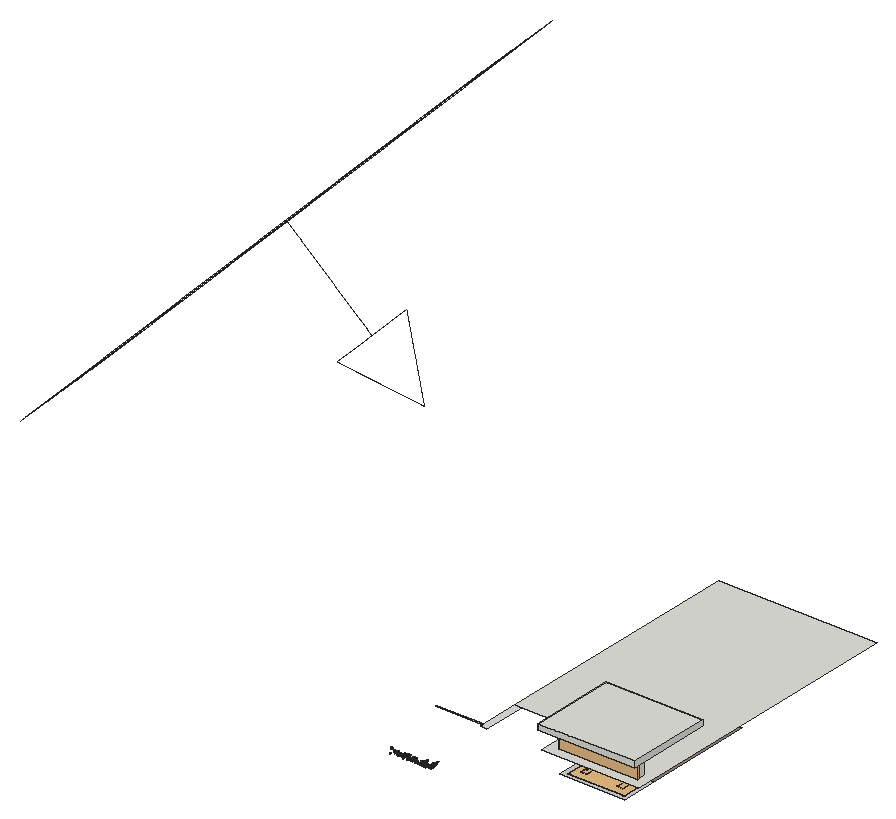
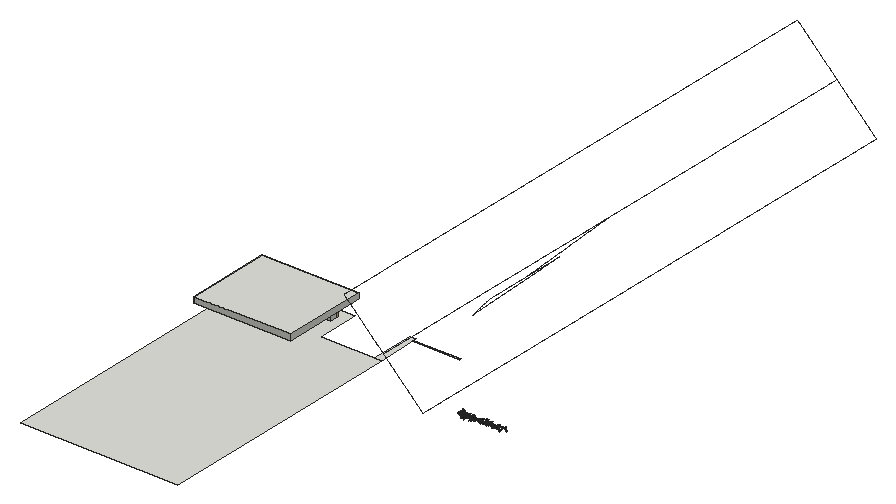
# SketchUp Ruby script. Lengths in inches.
U = 1.inch
M = Sketchup.active_model
def pt(a) = Geom::Point3d.new(a.map { |v| v * U })
def face(e, loops, mat)
  f = e.add_face(loops[0].map { |a| pt(a) })
  loops[1..].each { |l| e.add_face(l.map { |a| pt(a) }).erase! }
  f.material = f.back_material = mat if mat
  f
end
# faces: each face lists its corners as indices into pts; further lists are holes
def faces(e, pts, list, mat = nil) = list.each { |f| face(e, (f[0].is_a?(Array) ? f : [f]).map { |l| l.map { |i| pts[i] } }, mat) }
# xy, xz, yz: faces in a plane at the given z, y or x. An outline is a flat list of corners, or four numbers for a rectangle; further outlines are holes
def ring(l) = l.size == 4 ? [[l[0], l[1]], [l[2], l[1]], [l[2], l[3]], [l[0], l[3]]] : l.each_slice(2).to_a
def flat(e, list, mat, &to3) = list.each { |f| face(e, (f[0].is_a?(Array) ? f : [f]).map { |l| ring(l).map { |u, v| to3.(u, v) } }, mat) }
def xy(e, z, list, mat = nil) = flat(e, list, mat) { |x, y| [x, y, z] }
def xz(e, y, list, mat = nil) = flat(e, list, mat) { |x, z| [x, y, z] }
def yz(e, x, list, mat = nil) = flat(e, list, mat) { |y, z| [x, y, z] }
def lines(e, pts, list) = list.each { |a, b| e.add_line(pt(pts[a]), pt(pts[b])) }
# prism: a flat outline (further loops are holes) pulled along v
def prism(e, loops, v, mat = nil)
  f = face(e, loops, mat); d = Geom::Vector3d.new(v.map { |x| x * U })
  f.pushpull(f.normal.samedirection?(d) ? d.length : -d.length)
end
def box(e, o, s, mat = nil) = prism(e, [[o, [o[0] + s[0], o[1], o[2]], [o[0] + s[0], o[1] + s[1], o[2]], [o[0], o[1] + s[1], o[2]]]], [0, 0, s[2]], mat)
def at(x, y, z, deg = 0) = Geom::Transformation.translation(pt([x, y, z])) * Geom::Transformation.rotation(ORIGIN, Z_AXIS, deg.degrees)
def axes(o, x, y, z) = Geom::Transformation.new([*x, 0, *y, 0, *z, 0, *pt(o).to_a, 1])
def part(name) = M.definitions.add(name)
# library, detail: a bought-in or finely detailed component or shape, given as its bounding box
def library(name, o, s) = part(name).tap { |d| box(d.entities, o, s) }
def detail(e, o, s) = box(e.add_group.entities, o, s)
def put(e, d, t, mat = nil) = e.add_instance(d, t).tap { |i| i.material = mat if mat }
def group(e, t, mat = nil) = e.add_group.tap { |g| g.transformation = t; g.material = mat if mat }.entities
root = M.entities
M.materials.add("Concrete White 02 100cm").color = [209, 209, 209]
M.materials.add("Heather_Band").color = [140, 131, 120]
M.materials.add("efeu1").color = [18, 25, 13]
c1 = part("ivyleaf_9")
p = [[1.54,2.16,1.25],[1.36,2.04,1.19],[-0.21,0.99,0.68],[-0.71,1.11,0.82],[-0.85,0.86,0.67],[-0.8,0.17,0.21],
  [-0.9,-0.01,0.1],[-0.67,-0.16,-0.02],[-0.08,-0.08,-0.05],[-0.03,-0.6,-0.4],[0.65,-0.88,-0.66],[0.83,-0.6,-0.49],
  [1.29,-0.42,-0.43],[1.8125,-0.07,-0.26],[1.21,0.44,0.15]]
faces(c1.entities,p,[[0,1,2,3,4,5,6,7,8,9,10,11,12,13,14]],"efeu1")
c2 = library("Tlon Light 450 Ceiling 152 006",[-8.86,-8.86,-3.78],[17.72,17.72,3.56])
c3 = part("Tlon Cubo 860 Ceiling 152 005")
xy(c3.entities,-3.04,[[-16.54,-16.54,-16.54,16.54,16.54,-16.54],[16.54,-16.54,-16.54,16.54,16.54,16.54]])
xy(c3.entities,0,[[-16.93,-16.93,16.93,-16.93,-16.93,16.93],[16.93,-16.93,16.93,16.93,-16.93,16.93]])
xz(c3.entities,-16.93,[[-16.93,-3.79,16.93,-3.79,-16.93,0],[16.93,-3.79,16.93,0,-16.93,0]])
xz(c3.entities,-16.3,[[-16.3,-3.66,-16.3,-3.24,16.3,-3.24],[-16.3,-3.66,16.3,-3.24,16.3,-3.66]])
xz(c3.entities,16.3,[[-16.3,-3.66,16.3,-3.24,-16.3,-3.24],[-16.3,-3.66,16.3,-3.66,16.3,-3.24]])
xz(c3.entities,16.93,[[-16.93,-3.79,-16.93,0,16.93,0],[-16.93,-3.79,16.93,0,16.93,-3.79]])
yz(c3.entities,-16.93,[[-16.93,-3.79,-16.93,0,16.93,0],[-16.93,-3.79,16.93,0,16.93,-3.79]])
yz(c3.entities,-16.3,[[-16.3,-3.66,16.3,-3.66,-16.3,-3.24],[16.3,-3.66,16.3,-3.24,-16.3,-3.24]])
yz(c3.entities,16.3,[[-16.3,-3.66,-16.3,-3.24,16.3,-3.66],[16.3,-3.66,-16.3,-3.24,16.3,-3.24]])
yz(c3.entities,16.93,[[-16.93,-3.79,16.93,-3.79,-16.93,0],[16.93,-3.79,16.93,0,-16.93,0]])
p = [[-16.93,-16.93,-3.79],[-16.93,16.93,-3.79],[-16.3,16.3,-3.66],[-16.3,-16.3,-3.66],[16.93,-16.93,-3.79],[16.3,-16.3,-3.66],
  [16.93,16.93,-3.79],[16.3,16.3,-3.66]]
faces(c3.entities,p,[[0,1,2],[2,3,0],[4,0,3],[3,5,4],[6,4,5],[5,7,6],[2,1,6],[6,7,2]])
c4 = library("Group\#2",[-0.5,-0.5,-0.1],[76.5625,123.26,0.2])
c5 = library("Group\#11",[-0.5,-0.5,-0.1],[80.125,38.25,0.2])
c6 = library("Wall Panel 104-26",[-34.24,-2.8,0],[68.48,2.8,108.01])
c7 = part("Group418\#1")
p = [[0,0,0],[0,0,-140.58],[-66.03,0,-140.58],[429.86,-25.26,0],[-429.86,-25.26,0],[429.86,25.26,0],
  [429.86,0,0],[-429.86,25.26,0],[66.03,0,-140.58],[-429.86,0,0],[0,0,-227.5625]]
lines(c7.entities,p,[[0,1],[1,2],[3,4],[5,6],[7,5],[1,8],[9,0],[0,6],[8,10],[4,9],[6,3],[2,10],
  [9,7]])
c8 = part("Rectangle Light\#1")
put(c8.entities,c7,at(0,0,0))
xy(root,316.43,[[[245.01,223.4375,337.3,273.83],[252.75,229.09,331.875,266.34]],[254.75,231.09,329.875,264.34]],"Concrete White 02 100cm")
xy(root,316.43,[[[245.01,273.83,337.3,430.75],[253.2,286.86,328.77,409.125]],[255.2,288.86,326.77,407.125]],"Heather_Band")
xy(root,337.75,[[133.125,223.4375,142.16,284.3125],[[219.21,223.4375,356.8125,223.4375,356.8125,643.9375,133.125,643.9375,133.125,284.3125,219.21,284.3125],[232.57,240.26,343.51,249.58]],[66.5625,227.3125,133.125,229.125]])
xy(root,360.8,[[213.82,224.2,213.82,344.45,350.32,344.45,350.32,249.58,232.57,249.58,232.57,240.26,350.32,240.26,350.32,224.2],[232.57,240.26,343.51,249.58],[343.51,240.26,350.32,249.58]])
xy(root,369,[[213.82,224.2,350.32,344.45]])
xz(root,224.2,[[213.82,360.8,350.32,369]])
xz(root,240.26,[[232.57,337.75,343.51,360.8]])
xz(root,249.58,[[232.57,337.75,343.51,360.8]])
xz(root,344.45,[[213.82,360.8,350.32,369]])
yz(root,213.82,[[224.2,360.8,344.45,369]])
yz(root,232.57,[[240.26,337.75,249.58,360.8]])
yz(root,343.51,[[240.26,337.75,249.58,360.8]])
yz(root,350.32,[[224.2,360.8,344.45,369]])
put(root,c1,axes([54.86,220.23,262.29],[-0.42599,-0.23908,0.10667],[-0.08419,-0.0678,-0.48818],[0.24789,-0.43387,0.01751]))
put(root,c1,axes([54.96,223.33,262.27],[-0.42097,0.2695,0.0124],[-0.06704,-0.08224,-0.48861],[-0.26132,-0.41304,0.10537]))
put(root,c1,axes([44.03,219.59,262.4],[0.30234,-0.38809,-0.08932],[-0.02728,0.0917,-0.49076],[0.3973,0.30163,0.03428]))
put(root,c1,axes([64.83,220.53,262.52],[0.41955,-0.2121,-0.17026],[-0.05677,0.2378,-0.43615],[0.26599,0.38531,0.17546]))
put(root,c1,axes([27.72,218.6,262.27],[-0.41659,-0.27335,0.04161],[-0.03507,-0.0224,-0.49827],[0.27426,-0.41807,-0.00051]))
put(root,c1,axes([61.34,220.32,262.58],[0.1176,-0.43666,-0.2133],[0.00401,0.22032,-0.44883],[0.48596,0.10386,0.05533]))
put(root,c1,axes([53.86,220.5,262.4],[-0.38441,0.31571,-0.05054],[0.02059,-0.05442,-0.4966],[-0.31907,-0.38388,0.02884]))
put(root,c1,axes([34.49,220.18,262.66],[0.1015,-0.41881,-0.25356],[0.06389,0.26807,-0.4172],[0.4854,0.05229,0.10793]))
put(root,c1,axes([62.25,220.75,262.43],[0.28877,-0.40492,-0.05146],[0.01714,0.07502,-0.49404],[0.40782,0.28357,0.05721]))
put(root,c1,axes([54.6875,218.44,262.05],[0.04231,-0.15687,0.47286],[0.35975,-0.31869,-0.13791],[0.34466,0.35189,0.08591]))
put(root,c1,axes([64.3,220.32,262.65],[-0.06335,-0.43846,-0.23183],[0.04191,0.22814,-0.44294],[0.4942,-0.07555,0.00785]))
put(root,c1,axes([16.375,220.87,262.39],[0.02361,0.49902,-0.02055],[-0.00029,-0.02056,-0.49958],[-0.49944,0.0236,-0.00068]))
put(root,c1,axes([42.61,220.58,262.42],[0.44072,-0.22677,0.06591],[0.05993,-0.02758,-0.49563],[0.22842,0.44476,0.00287]))
put(root,c1,axes([51.43,220.61,262.45],[-0.04152,-0.48791,0.10112],[-0.01245,-0.10042,-0.48965],[0.49812,-0.04318,-0.00381]))
put(root,c1,axes([62.4,220.6875,262.71],[0.00392,-0.30471,-0.39641],[0.18464,0.36928,-0.28203],[0.46464,-0.14417,0.11542]))
put(root,c1,axes([27.24,219.85,262.5],[-0.41595,0.06259,0.27031],[-0.27588,-0.04138,-0.41495],[-0.02957,-0.49434,0.06895]))
put(root,c1,axes([62.33,220.75,262.4],[0.00894,-0.49992,0.00077],[-0.00005,-0.00077,-0.5],[0.49992,0.00894,-0.00006]))
put(root,c1,axes([32.43,219.17,262.8],[0.22625,-0.3949,-0.20703],[-0.01221,0.22658,-0.44555],[0.44571,0.20667,0.09288]))
put(root,c1,axes([54.54,220.27,262.72],[-0.21236,0.04329,-0.45059],[0.39361,-0.22814,-0.20742],[-0.22355,-0.44281,0.06282]))
put(root,c1,axes([26.86,220.45,262.53],[-0.14827,-0.47751,0.00136],[0.00832,-0.00401,-0.49991],[0.47744,-0.14822,0.00913]))
put(root,c1,axes([63.24,220.27,262.65],[0.13031,0.42767,0.22387],[-0.04054,0.24076,-0.43634],[-0.48102,0.09557,0.09742]))
put(root,c1,axes([52.2,219.52,262.55],[-0.1899,0.28378,0.36525],[-0.22412,0.28893,-0.34101],[-0.40461,-0.29323,0.01747]))
put(root,c1,axes([44.57,218.84,262.68],[-0.23037,-0.41187,0.1652],[-0.02076,-0.17593,-0.46757],[0.44328,-0.22229,0.06396]))
put(root,c1,axes([51.34,219.01,262.74],[-0.26364,-0.41336,0.09811],[-0.00422,-0.11291,-0.48707],[0.42482,-0.25765,0.05605]))
put(root,c1,axes([55.45,222.27,262.38],[0.19075,-0.44838,0.11209],[0.43896,0.13781,-0.19575],[0.14465,0.17309,0.44622]))
put(root,c1,axes([62.76,220.68,262.04],[0.00862,-0.49987,-0.00733],[-0.0052,-0.00742,0.49992],[-0.4999,-0.00854,-0.00532]))
put(root,c1,axes([65.45,220.93,262.85],[-0.32857,-0.36504,-0.09375],[0.09576,0.03944,-0.48916],[0.36452,-0.3394,0.044]))
put(root,c1,axes([24.79,220.5,262.8125],[-0.39253,-0.27217,0.14781],[-0.03644,-0.19638,-0.45837],[0.30756,-0.37062,0.13434]))
put(root,c1,axes([59.54,220.23,263.04],[0.18927,-0.36787,-0.28079],[-0.05174,0.28465,-0.4078],[0.45989,0.18342,0.06968]))
put(root,c1,axes([25.62,220.68,262.78],[-0.14463,-0.46314,0.12077],[0.00539,-0.12773,-0.48338],[0.4786,-0.13852,0.04194]))
put(root,c1,axes([50.69,221.84,262.58],[-0.09558,-0.47416,0.12664],[0.38768,-0.15206,-0.27673],[0.30094,0.04529,0.39671]))
put(root,c1,axes([45.11,219.73,262.8125],[-0.23768,-0.3743,0.2311],[-0.05756,-0.23395,-0.43812],[0.43611,-0.23487,0.06812]))
put(root,c1,axes([59.52,219.48,262.73],[-0.28352,-0.41013,0.03755],[-0.01761,-0.03347,-0.49857],[0.41147,-0.28403,0.00454]))
put(root,c1,axes([56.01,220.41,262.85],[-0.32635,-0.35473,0.13289],[0.00327,-0.17803,-0.46722],[0.37879,-0.30409,0.11852]))
put(root,c1,axes([54.41,220.22,262.8],[0.33289,-0.35914,0.10102],[0.06557,-0.07696,-0.48967],[0.36727,0.33926,-0.00415]))
put(root,c1,axes([62.76,220.74,263.01],[0.02708,-0.45074,-0.21471],[-0.01048,0.21446,-0.45155],[0.49916,0.02896,0.00217]))
put(root,c1,axes([51.44,220.54,262.78],[-0.46496,-0.18005,0.03741],[-0.02623,-0.03575,-0.49803],[0.18201,-0.46509,0.0238]))
put(root,c1,axes([53.25,220.42,262.83],[-0.39244,-0.30546,-0.05179],[0.03661,0.03728,-0.49726],[0.30765,-0.39409,-0.00689]))
put(root,c1,axes([53.93,220.66,262.75],[0.49126,0.09289,0.00575],[0.00553,0.00172,-0.49997],[-0.0929,0.49129,0.00066]))
put(root,c1,axes([57.3125,217.79,262.8],[-0.05606,-0.38295,0.31655],[-0.0145,-0.31716,-0.38626],[0.49664,-0.05249,0.02446]))
put(root,c1,axes([57.07,220.22,263.01],[0.48447,0.02247,-0.1216],[-0.12366,0.08909,-0.47621],[0.00026,0.49149,0.09188]))
put(root,c1,axes([37.4375,220.05,263.05],[-0.01349,-0.47015,-0.16962],[0.03219,0.16852,-0.46964],[0.49878,-0.02359,0.02572]))
put(root,c1,axes([63.16,220.43,262.88],[0.35063,-0.34155,0.102],[0.06068,-0.0838,-0.48918],[0.35125,0.35542,-0.01731]))
put(root,c1,axes([48.5,219.26,262.89],[0.03823,-0.43681,0.24028],[0.0167,-0.23973,-0.43847],[0.49826,0.04155,-0.00374]))
put(root,c1,axes([56.67,220.22,263.125],[0.21117,0.22936,-0.3909],[-0.28869,-0.26436,-0.31108],[-0.34938,0.35708,0.02078]))
put(root,c1,axes([34.86,220.57,262.9],[0.44413,-0.21171,0.08904],[0.09128,-0.01518,-0.49136],[0.21075,0.45271,0.02517]))
put(root,c1,axes([9.25,217.91,262.78],[-0.01293,-0.09978,-0.48977],[0.48915,0.09822,-0.03292],[0.10279,-0.48,0.09507]))
put(root,c1,axes([34.9,220.8,262.95],[-0.20847,0.45265,0.04063],[-0.10565,-0.00479,-0.48869],[-0.44201,-0.21234,0.09765]))
put(root,c1,axes([26.57,220.6,262.94],[0.28714,0.40359,0.0683],[0.03646,0.05788,-0.4953],[-0.4077,0.28942,0.0038]))
put(root,c1,axes([39.71,220.23,262.9375],[-0.11352,-0.48636,-0.02387],[0.0055,0.02323,-0.49943],[0.48691,-0.11365,0.00008]))
put(root,c1,axes([25.39,220.45,262.97],[0.08966,-0.49004,-0.04264],[-0.00513,0.0424,-0.49817],[0.49187,0.08977,0.00258]))
put(root,c1,axes([44.56,220.14,263.23],[0.04803,-0.39539,-0.30226],[-0.02594,0.30126,-0.39821],[0.49701,0.05394,0.00843]))
put(root,c1,axes([45.04,219.96,262.97],[-0.03968,-0.49059,0.08801],[-0.01222,-0.0873,-0.49217],[0.49827,-0.0412,-0.00506]))
put(root,c1,axes([66.34,219.49,263.18],[-0.1006,0.4545,-0.1825],[0.00056,-0.1862,-0.46403],[-0.48977,-0.09357,0.03695]))
put(root,c1,axes([65.85,220.65,262.96],[-0.06197,-0.49556,-0.02414],[0.00298,0.02395,-0.49942],[0.49614,-0.06204,-0.00002]))
put(root,c1,axes([27.74,220.67,263.03],[-0.15866,0.4626,0.10408],[-0.01791,0.10383,-0.48877],[-0.47382,-0.15883,-0.01638]))
put(root,c1,axes([45.53,218.7,263.07],[-0.23,-0.40771,0.1757],[-0.02789,-0.18422,-0.46399],[0.44308,-0.22324,0.062]))
put(root,c1,axes([55.13,223.34,262.99],[0.11409,0.48651,-0.01699],[0.00618,-0.01889,-0.4996],[-0.48677,0.11379,-0.01033]))
put(root,c1,axes([49.55,219.02,263.08],[0.06823,-0.47415,0.14328],[0.06541,-0.13474,-0.47704],[0.49099,0.08384,0.04364]))
put(root,c1,axes([27.18,220.61,263.01],[-0.12734,-0.4835,0.00349],[0.00549,-0.00506,-0.49994],[0.48348,-0.12728,0.0066]))
put(root,c1,axes([48.39,219.68,263.08],[0.07777,-0.4905,0.058],[0.02213,-0.05519,-0.49645],[0.49342,0.07979,0.01313]))
put(root,c1,axes([45.74,220.05,263.25],[0.48177,-0.06143,-0.11884],[-0.11061,0.0669,-0.483],[0.07524,0.49168,0.05088]))
put(root,c1,axes([63.73,220.83,263.09],[-0.00171,-0.49985,-0.01222],[-0.01811,0.01228,-0.49952],[0.49967,-0.00127,-0.01815]))
put(root,c1,axes([60.8,220.35,263.12],[-0.44271,-0.23214,-0.01101],[0.03615,-0.04539,-0.49662],[0.22958,-0.44051,0.05697]))
put(root,c1,axes([64.61,220.28,263.21],[0.00194,-0.49595,-0.06346],[0.04684,0.06337,-0.49375],[0.4978,-0.00403,0.04671]))
put(root,c1,axes([37.23,219.53,263.22],[-0.11113,-0.4265,0.23612],[0.03115,-0.24789,-0.4331],[0.4865,-0.08155,0.08167]))
put(root,c1,axes([57.37,218.68,263.34],[-0.16549,0.44855,-0.14634],[0.02887,-0.14516,-0.47759],[-0.47093,-0.16653,0.02215]))
put(root,c1,axes([23.6875,220.43,263.31],[-0.17531,-0.45624,-0.10542],[0.02482,0.10336,-0.48857],[0.4676,-0.17653,-0.01359]))
put(root,c1,axes([19.4375,218.25,263.52],[0.37634,-0.18839,-0.26996],[-0.1736,0.2348,-0.40587],[0.27969,0.39922,0.11132]))
put(root,c1,axes([57.42,219.74,263.2],[0.29389,-0.40307,0.03414],[0.0193,-0.02818,-0.49883],[0.40405,0.29452,-0.001]))
put(root,c1,axes([55.92,219.93,263.2],[-0.25571,-0.17363,0.39302],[-0.20705,-0.35095,-0.28976],[0.37648,-0.31094,0.10758]))
put(root,c1,axes([51.95,222.1875,262.92],[0.44905,-0.15697,-0.154],[0.13646,0.4735,-0.08472],[0.17244,0.03406,0.46809]))
put(root,c1,axes([56.91,220.37,263.26],[-0.19296,-0.46117,-0.00935],[0.00475,0.00814,-0.49991],[0.46124,-0.19301,0.00124]))
put(root,c1,axes([59.51,220.4,263.26],[-0.37773,0.32754,0.00626],[-0.00506,0.00373,-0.49996],[-0.32756,-0.37776,0.0005]))
put(root,c1,axes([55.69,224.26,263.35],[0.46805,-0.16836,-0.05084],[-0.04404,0.02774,-0.49728],[0.17027,0.46998,0.01114]))
put(root,c1,axes([46.15,218.59,263.45],[-0.2698,-0.38429,0.17183],[-0.02844,-0.18699,-0.46285],[0.42,-0.25953,0.07904]))
put(root,c1,axes([47.38,218.45,263.46],[0.02221,-0.49075,0.09314],[0.01411,-0.09258,-0.49115],[0.49931,0.02445,0.00974]))
put(root,c1,axes([49.75,218.87,263.59],[-0.09108,-0.47565,-0.12433],[0.01252,0.12416,-0.48418],[0.49148,-0.09131,-0.01071]))
put(root,c1,axes([55.82,223.97,263.6],[-0.35277,0.33745,-0.1081],[0.04656,-0.10707,-0.48618],[-0.35127,-0.35308,0.04412]))
put(root,c1,axes([63.125,225.89,263.42],[-0.09344,0.49113,-0.00784],[0.00142,-0.00771,-0.49994],[-0.49119,-0.09346,0.00004]))
put(root,c1,axes([60.78,220.4,262.92],[0.04504,-0.11242,0.48511],[-0.17636,0.45192,0.1211],[-0.46569,-0.18202,0.00106]))
put(root,c1,axes([64.38,220.39,263.61],[0.3924,-0.20854,0.2292],[0.23881,-0.03215,-0.43811],[0.19746,0.4533,0.07437]))
put(root,c1,axes([13.99,220.84,263.53],[-0.19403,-0.46014,0.02498],[-0.007,-0.02416,-0.49937],[0.46076,-0.19413,0.00293]))
put(root,c1,axes([54.82,220.36,263.67],[0.09333,-0.48372,-0.08545],[-0.00899,0.08528,-0.49259],[0.49113,0.09348,0.00722]))
put(root,c1,axes([66.21,226.25,263.6],[-0.48799,-0.069,0.08429],[-0.08122,-0.02734,-0.4926],[0.07259,-0.49446,0.01548]))
put(root,c1,axes([65.76,220.78,263.29],[-0.15891,0.08283,0.46678],[-0.40599,0.23042,-0.1791],[-0.24478,-0.43594,-0.00597]))
put(root,c1,axes([44.97,220.39,263.67],[-0.16115,-0.46869,-0.06599],[0.0231,0.06184,-0.49562],[0.47275,-0.16279,0.00172]))
put(root,c1,axes([56.28,217.98,263.9],[-0.05485,-0.41106,-0.27932],[0.06141,0.27326,-0.4142],[0.49317,-0.07974,0.02051]))
put(root,c1,axes([27.27,220.42,263.67],[-0.27658,-0.40573,0.09429],[0.01018,-0.11974,-0.48534],[0.41642,-0.26655,0.07449]))
put(root,c1,axes([21.9375,219.99,263.61],[0.0833,-0.49203,0.03114],[0.00099,-0.03141,-0.49901],[0.49301,0.0832,-0.00426]))
put(root,c1,axes([62.93,220.4,263.48],[0.31579,-0.14652,-0.3589],[0.33162,-0.13762,0.34798],[-0.20075,-0.45781,0.01026]))
put(root,c1,axes([53.41,219.87,263.61],[-0.2446,-0.43608,0.00133],[0.00908,-0.00662,-0.49987],[0.43599,-0.24451,0.01116]))
put(root,c1,axes([55.29,222.23,263.43],[-0.45541,-0.15717,0.1338],[0.08574,-0.43887,-0.22371],[0.18776,-0.18081,0.42667]))
put(root,c1,axes([65.01,220.77,263.58],[0.27946,-0.15529,0.38443],[0.33781,-0.18351,-0.3197],[0.24039,0.43842,0.00234]))
put(root,c1,axes([40.92,220.48,263.71],[-0.05558,-0.49234,0.06716],[-0.00043,-0.06753,-0.49542],[0.4969,-0.05513,0.00708]))
put(root,c1,axes([28.29,220.46,263.86],[0.36282,-0.33061,-0.0952],[0.00965,0.14808,-0.47747],[0.3439,0.34463,0.11384]))
put(root,c1,axes([43.09,220,263.83],[-0.26637,0.41511,-0.08201],[0.04853,-0.06629,-0.4932],[-0.42034,-0.27071,-0.00498]))
put(root,c1,axes([64.75,220.07,263.73],[-0.28076,0.41331,-0.01865],[0.01108,-0.01502,-0.49965],[-0.41358,-0.28098,-0.00073]))
put(root,c1,axes([27.97,220.71,263.78],[-0.31824,0.38268,0.04774],[-0.07449,-0.00026,-0.49442],[-0.37838,-0.3218,0.05718]))
put(root,c1,axes([21.72,220.45,263.87],[-0.27275,-0.40808,0.0953],[0.03251,-0.13397,-0.48062],[0.41779,-0.25598,0.09962]))
put(root,c1,axes([22.6,220.4,263.92],[0.10321,-0.48284,-0.0788],[0.00389,0.08134,-0.49332],[0.48922,0.10122,0.02054]))
put(root,c1,axes([66.41,220.47,263.9],[0.21563,-0.44804,-0.05258],[-0.01138,0.05286,-0.49707],[0.45097,0.21556,0.0126]))
put(root,c1,axes([26.76,220.6875,263.89],[-0.0398,0.49745,-0.03095],[0.00673,-0.03051,-0.49902],[-0.49837,-0.04014,-0.00427]))
put(root,c1,axes([62.99,220.55,263.87],[-0.04029,-0.49827,-0.01018],[-0.01516,0.01143,-0.49964],[0.49814,-0.03995,-0.01602]))
put(root,c1,axes([43.48,220.27,263.88],[-0.34092,-0.36574,0.00233],[-0.00926,0.00545,-0.49988],[0.36563,-0.34089,-0.01049]))
put(root,c1,axes([20.36,220.62,263.56],[0.11577,0.08062,0.47969],[0.33546,0.34383,-0.13875],[-0.35223,0.35395,0.02553]))
put(root,c1,axes([27.65,220.26,264.03],[-0.06263,0.47858,0.13054],[-0.11996,0.11306,-0.47204],[-0.48134,-0.09045,0.10066]))
put(root,c1,axes([56.68,219.78,264.07],[0.47041,0.15013,-0.07858],[-0.06916,-0.04157,-0.49345],[-0.15469,0.47512,-0.01834]))
put(root,c1,axes([20.6875,220.4375,264.28],[0.37399,0.11656,-0.31072],[-0.31547,-0.02047,-0.38738],[-0.10303,0.48579,0.05823]))
put(root,c1,axes([43.09,220.32,264.04],[0.09511,-0.48795,-0.05346],[0.01428,0.05718,-0.49651],[0.49066,0.09292,0.02481]))
put(root,c1,axes([45.37,220.71,264.03],[0.33445,0.35584,0.10735],[0.05121,0.09892,-0.48743],[-0.36813,0.33704,0.02972]))
put(root,c1,axes([31.33,220.63,264.27],[-0.08832,-0.43031,-0.23882],[0.09772,0.22247,-0.43698],[0.48234,-0.12386,0.0448]))
put(root,c1,axes([27.65,219.58,264.08],[-0.42734,-0.25695,-0.0369],[0.03966,0.00561,-0.49839],[0.25654,-0.42889,0.01559]))
put(root,c1,axes([45.5,219.93,264.04],[-0.02444,-0.4994,0.00141],[-0.00798,-0.00102,-0.49994],[0.49934,-0.02446,-0.00792]))
put(root,c1,axes([65.46,226.26,264.11],[0.49977,-0.01513,0.00069],[0.0007,0.0006,-0.5],[0.01513,0.49977,0.00062]))
put(root,c1,axes([63.4,225.93,264.28],[0.38119,0.24332,0.21328],[0.17006,0.12972,-0.45194],[-0.27527,0.41709,0.01614]))
put(root,c1,axes([42.22,220.32,263.96],[0.14086,0.1077,0.4675],[0.27422,0.38172,-0.17056],[-0.39365,0.30445,0.04847]))
put(root,c1,axes([66.74,226.3125,264.48],[-0.27439,0.38213,-0.16938],[0.06905,-0.15839,-0.4692],[-0.41224,-0.28088,0.03415]))
put(root,c1,axes([65.37,219.42,264.52],[-0.40305,-0.21563,-0.20262],[0.19069,0.07252,-0.45649],[0.22625,-0.44525,0.02377]))
put(root,c1,axes([54.56,220.24,264.3],[0.45211,-0.21308,-0.0141],[0.0208,0.07679,-0.49363],[0.21253,0.44576,0.07829]))
put(root,c1,axes([68.75,220.32,264.58],[-0.26554,-0.22666,-0.35793],[0.27031,0.23463,-0.34912],[0.32622,-0.37891,-0.00206]))
put(root,c1,axes([64.1,220.68,264.42],[-0.47206,-0.07064,0.1489],[-0.14122,-0.05949,-0.47594],[0.08495,-0.4914,0.03621]))
put(root,c1,axes([17.44,219.82,264.57],[0.15104,-0.45741,-0.13401],[0.01497,0.14506,-0.47826],[0.47641,0.14046,0.05751]))
put(root,c1,axes([35.73,219.71,264.7],[-0.08329,-0.33989,-0.35713],[0.27789,0.2668,-0.31874],[0.40723,-0.25158,0.14446]))
put(root,c1,axes([67.35,219.4,264.42],[-0.18967,-0.45962,0.05271],[-0.02848,-0.04526,-0.49713],[0.46175,-0.19158,-0.00901]))
put(root,c1,axes([64.64,220.6875,264.35],[0.04035,-0.02038,-0.49795],[0.47205,-0.15865,0.04475],[-0.15983,-0.47372,0.00643]))
put(root,c1,axes([63.46,218.97,264.54],[-0.46408,0.18264,0.03561],[-0.02688,0.02888,-0.49844],[-0.18413,-0.46455,-0.01699]))
put(root,c1,axes([36.98,219.03,264.52],[0.20364,-0.4563,0.01794],[0.00587,-0.01702,-0.49968],[0.45661,0.20372,-0.00157]))
put(root,c1,axes([57.17,218.91,264.87],[-0.42729,0.01343,-0.25931],[0.24483,-0.14551,-0.41096],[-0.0865,-0.47817,0.11777]))
put(root,c1,axes([66.46,226.36,264.82],[-0.43962,0.13027,-0.1994],[0.16361,-0.13905,-0.45155],[-0.1731,-0.46227,0.07963]))
put(root,c1,axes([20.81,220.37,264.85],[-0.1859,-0.41159,-0.21456],[0.08097,0.19882,-0.45157],[0.45704,-0.20264,-0.00727]))
put(root,c1,axes([66.87,220.34,264.7],[0.19495,-0.45309,-0.08186],[-0.01834,0.08119,-0.49302],[0.46006,0.19524,0.01504]))
put(root,c1,axes([44.17,220.04,264.68],[-0.22002,-0.39127,0.22022],[-0.0612,-0.21681,-0.44637],[0.4448,-0.22338,0.04751]))
put(root,c1,axes([36.03,219.62,264.79],[0.09041,-0.47363,-0.13231],[0.00072,0.13465,-0.48153],[0.49176,0.08688,0.02503]))
put(root,c1,axes([36.04,220.63,264.8],[0.27078,-0.40452,-0.1142],[0.00144,0.13674,-0.48094],[0.42033,0.26013,0.07522]))
put(root,c1,axes([54.11,220.28,264.8125],[-0.20779,0.43863,-0.1201],[0.04373,-0.11216,-0.48529],[-0.45267,-0.21219,0.00825]))
put(root,c1,axes([31.19,220.71,264.87],[0.31174,-0.3782,-0.09892],[0.01509,0.13807,-0.48032],[0.39063,0.29649,0.0975]))
put(root,c1,axes([34.46,219.8125,264.77],[0.43009,-0.19732,0.16152],[0.14857,-0.0635,-0.47318],[0.20725,0.45501,0.00401]))
put(root,c1,axes([57.47,220.01,264.47],[-0.0602,0.1628,0.4689],[-0.22554,0.41179,-0.17193],[-0.44216,-0.23222,0.02386]))
put(root,c1,axes([30.73,220.3,264.96],[-0.05838,-0.47522,-0.14409],[0.01291,0.14358,-0.47877],[0.49641,-0.05962,-0.0045]))
put(root,c1,axes([56.61,219.24,265.03],[-0.41042,-0.21659,-0.18613],[0.17501,0.06675,-0.46359],[0.22567,-0.44568,0.02102]))
put(root,c1,axes([24.38,220.23,264.88],[-0.06246,-0.44627,0.21665],[0.03189,-0.22152,-0.44711],[0.49506,-0.04203,0.05614]))
put(root,c1,axes([53.51,220.45,265.09],[0.08719,-0.43172,-0.23668],[-0.01635,0.23769,-0.43959],[0.49207,0.08439,0.02733]))
put(root,c1,axes([59.47,220.15,264.85],[-0.12495,-0.48272,-0.03702],[0.00607,0.03666,-0.49862],[0.4841,-0.12505,-0.0033]))
put(root,c1,axes([55.66,223.16,264.97],[0.09678,0.48479,-0.07493],[-0.07704,-0.06041,-0.49032],[-0.48446,0.10645,0.063]))
put(root,c1,axes([67.34,220.59,265.07],[0.01259,-0.47317,-0.16111],[0.00675,0.16131,-0.47322],[0.4998,0.00974,0.01045]))
put(root,c1,axes([26.09,220.48,265.06],[0.02003,-0.4755,-0.15329],[-0.00253,0.15332,-0.47591],[0.49959,0.01984,0.00374]))
put(root,c1,axes([41.77,220.44,264.96],[-0.2914,0.33089,0.23578],[-0.20428,0.1315,-0.43701],[-0.35122,-0.35102,0.05855]))
put(root,c1,axes([19.13,218.8125,265],[-0.43976,-0.14129,0.19144],[-0.13634,-0.18006,-0.44608],[0.195,-0.44454,0.11984]))
put(root,c1,axes([20.32,220.21,264.98],[0.02087,-0.48565,0.11707],[0.02452,-0.11603,-0.48573],[0.49896,0.02601,0.01897]))
put(root,c1,axes([55.76,223.48,265.24],[-0.40206,0.1132,-0.27483],[0.26197,-0.08347,-0.41762],[-0.14043,-0.47981,0.00781]))
put(root,c1,axes([65.53,218.11,265.01],[-0.2507,-0.42977,-0.04949],[0.02983,0.03989,-0.49751],[0.43158,-0.2524,0.00564]))
put(root,c1,axes([28.43,220.48,264.98],[0.49935,0.0254,0.00094],[-0.00388,0.09436,-0.491],[-0.02512,0.49036,0.09444]))
put(root,c1,axes([53.85,220.13,265.04],[-0.25239,0.41683,0.11206],[-0.08777,0.07753,-0.48609],[-0.42261,-0.26504,0.03403]))
put(root,c1,axes([65.08,220.67,264.96],[0.03026,-0.49894,0.01202],[0.00014,-0.01203,-0.49986],[0.49908,0.03026,-0.00059]))
put(root,c1,axes([28.53,220.26,265.06],[0.01793,-0.4829,0.12841],[-0.00131,-0.12854,-0.48319],[0.49968,0.01699,-0.00587]))
put(root,c1,axes([37.26,220.14,265.01],[0.10375,0.48811,0.03146],[-0.00656,0.03354,-0.49883],[-0.48907,0.10309,0.01337]))
put(root,c1,axes([66.78,217.58,265.06],[-0.48131,0.12887,0.04169],[-0.04255,0.00225,-0.49818],[-0.12859,-0.4831,0.0088]))
put(root,c1,axes([12.96,220.66,265.34],[0.18632,-0.40791,-0.22113],[-0.04297,0.2221,-0.4459],[0.462,0.18516,0.04771]))
put(root,c1,axes([21.5625,220.29,265.25],[-0.10629,-0.46585,-0.14726],[0.04251,0.14131,-0.47773],[0.48672,-0.11407,0.00957]))
put(root,c1,axes([65.37,220.6,265.29],[-0.15692,-0.46216,-0.10857],[0.01766,0.10858,-0.48775],[0.47441,-0.15691,-0.01775]))
put(root,c1,axes([50.8125,220.46,265.44],[0.0259,-0.4596,-0.19519],[-0.00702,0.19509,-0.46031],[0.49928,0.02658,0.00365]))
put(root,c1,axes([67.67,220.44,265.14],[0.29001,-0.09734,0.3955],[0.38056,-0.10826,-0.3057],[0.14515,0.47834,0.0113]))
put(root,c1,axes([66.88,220.6,265.3],[-0.28294,0.28323,0.29955],[-0.21401,0.20961,-0.40033],[-0.35234,-0.35475,0.00261]))
put(root,c1,axes([20.96,220.31,265.4],[0.06417,-0.49027,-0.07426],[0.04123,0.07989,-0.49185],[0.49415,0.057,0.05068]))
put(root,c1,axes([65.58,220.32,265.58],[0.15249,-0.43317,-0.19776],[-0.00687,0.20563,-0.45571],[0.47613,0.1417,0.05676]))
put(root,c1,axes([19.5,219.34,265.19],[0.02541,0.26118,0.42561],[-0.23377,0.38279,-0.22095],[-0.44125,-0.18776,0.14156]))
put(root,c1,axes([27.98,220.53,265.46],[0.15119,-0.42367,0.21829],[0.12735,-0.18477,-0.44681],[0.45927,0.1907,0.05203]))
put(root,c1,axes([64.86,219.71,265.61],[0.21386,-0.10901,-0.43861],[-0.3399,0.28103,-0.23557],[0.29789,0.39892,0.04609]))
put(root,c1,axes([66.44,219.91,265.65],[0.4496,0.13666,-0.17084],[-0.17347,-0.01522,-0.46869],[-0.13331,0.48072,0.03373]))
put(root,c1,axes([34.8125,220.625,265.56],[-0.14865,-0.47631,-0.03206],[0.00844,0.03094,-0.49897],[0.47732,-0.14889,-0.00116]))
put(root,c1,axes([42.61,220.34,265.64],[-0.29652,-0.31353,0.25253],[-0.01201,-0.30661,-0.39477],[0.40241,-0.24018,0.1743]))
put(root,c1,axes([66.82,226.24,265.88],[0.08201,-0.41462,-0.26714],[0.03098,0.2746,-0.4167],[0.49225,0.0518,0.07073]))
put(root,c1,axes([67.38,219.26,265.74],[-0.25863,-0.41919,-0.086],[0.04004,0.07634,-0.49251],[0.42604,-0.26164,-0.00592]))
put(root,c1,axes([27.9,220.08,265.71],[-0.09578,-0.47121,0.13708],[0.01479,-0.14238,-0.47907],[0.49052,-0.08771,0.04121]))
put(root,c1,axes([28.09,219.77,265.65],[-0.49475,0.07025,-0.017],[0.01761,0.00308,-0.49968],[-0.0701,-0.49503,-0.00552]))
put(root,c1,axes([19.72,218.9375,265.71],[-0.48195,-0.00215,0.1331],[-0.13311,0.0142,-0.48175],[-0.00171,-0.49979,-0.01426]))
put(root,c1,axes([28.64,220.3,265.85],[0.4065,0.25171,-0.14628],[-0.13881,-0.05325,-0.47739],[-0.25591,0.42873,0.02658]))
put(root,c1,axes([54.13,219.62,265.72],[-0.33848,-0.28338,0.23479],[-0.18584,-0.14371,-0.44137],[0.31763,-0.38606,-0.00804]))
put(root,c1,axes([61.54,218.14,265.7],[0.02607,-0.49928,-0.00624],[-0.0005,0.00623,-0.49996],[0.49932,0.02608,-0.00017]))
put(root,c1,axes([28.89,220.4,265.88],[-0.12363,-0.47484,-0.09616],[0.00853,0.09709,-0.49041],[0.4844,-0.1229,-0.01591]))
put(root,c1,axes([28.8125,220.44,265.95],[-0.14081,-0.47651,0.05576],[0.08468,-0.08189,-0.48593],[0.47223,-0.1274,0.10376]))
put(root,c1,axes([65.89,225.88,265.89],[-0.38957,0.31299,-0.01641],[0.01227,-0.01093,-0.49973],[-0.31318,-0.38976,0.00083]))
put(root,c1,axes([40.44,219.91,266.16],[-0.30776,-0.35933,0.16175],[0.01949,-0.21886,-0.44913],[0.39358,-0.27015,0.14872]))
put(root,c1,axes([61.39,218.29,266.24],[-0.41909,-0.11722,0.24621],[-0.20327,-0.16663,-0.42534],[0.18177,-0.45661,0.09201]))
put(root,c1,axes([41.49,219.875,266.41],[-0.11594,-0.44989,-0.18482],[0.05802,0.17585,-0.46445],[0.4829,-0.12915,0.01143]))
put(root,c1,axes([68.12,220.42,266.23],[-0.35141,0.35511,-0.02021],[0.01024,-0.0183,-0.49956],[-0.35554,-0.35152,0.00559]))
put(root,c1,axes([67.57,220.53,266.62],[0.20397,-0.35766,-0.28369],[-0.13418,0.25002,-0.41169],[0.43634,0.24407,0.00601]))
put(root,c1,axes([56.41,224.85,266.66],[0.12961,-0.40184,-0.26781],[-0.04296,0.2666,-0.42081],[0.48099,0.13209,0.03458]))
put(root,c1,axes([66.26,220.17,266.49],[0.0166,0.49261,-0.08402],[-0.02592,-0.08311,-0.49236],[-0.49905,0.0207,0.02278]))
put(root,c1,axes([68.3,226.22,266.71],[-0.14827,-0.25458,-0.40398],[0.31717,0.26371,-0.28259],[0.35695,-0.34007,0.08329]))
put(root,c1,axes([29.26,220.41,266.47],[-0.33313,-0.37169,0.02948],[0.0409,-0.07572,-0.49254],[0.37061,-0.32575,0.08086]))
put(root,c1,axes([29.68,220.24,266.75],[0.09675,-0.45172,-0.19128],[0.00086,0.19513,-0.46035],[0.49055,0.08875,0.03853]))
put(root,c1,axes([68.96,219.78,266.56],[0.41251,-0.28159,-0.0233],[0.05808,0.12485,-0.48067],[0.27652,0.39385,0.13571]))
put(root,c1,axes([31.51,218.83,266.79],[-0.10371,-0.43584,-0.222],[0.05739,0.21453,-0.44798],[0.48575,-0.1184,0.00553]))
put(root,c1,axes([55.65,223.34,266.67],[-0.20169,0.45336,-0.06154],[-0.04036,-0.08462,-0.49113],[-0.45573,-0.19315,0.07072]))
put(root,c1,axes([13.29,220.52,266.83],[0.20611,-0.41378,-0.19053],[-0.00038,0.20897,-0.45424],[0.45554,0.18739,0.08583]))
put(root,c1,axes([68.49,220.4,266.93],[-0.26262,-0.36012,-0.22659],[0.12278,0.19081,-0.44555],[0.40738,-0.28966,-0.0118]))
put(root,c1,axes([67.4,219.875,266.77],[0.45024,-0.13284,0.17215],[0.17957,0.00392,-0.46663],[0.12262,0.48202,0.05123]))
put(root,c1,axes([44.33,220.54,266.98],[-0.41673,-0.24456,-0.12857],[0.11017,0.0663,-0.48318],[0.25338,-0.43104,-0.00137]))
put(root,c1,axes([42.43,219.7,267],[-0.47456,-0.07899,0.1362],[-0.13513,-0.01761,-0.48107],[0.0808,-0.49341,-0.00464]))
put(root,c1,axes([67.21,219.87,266.96],[-0.21015,-0.45365,0.00597],[-0.00387,-0.00479,-0.49996],[0.45368,-0.21018,-0.0015]))
put(root,c1,axes([68.69,226.37,267.05],[-0.0022,0.49559,0.06623],[-0.02955,0.06598,-0.49475],[-0.49912,-0.00609,0.029]))
put(root,c1,axes([30.28,219.36,267.18],[0.15048,0.47236,-0.06505],[-0.156,-0.01568,-0.47478],[-0.45058,0.16319,0.14266]))
put(root,c1,axes([70.54,220.96,267.51],[-0.27974,0.38182,-0.16113],[0.04487,-0.16535,-0.46973],[-0.41199,-0.27726,0.05825]))
put(root,c1,axes([55.47,219.35,267.55],[-0.41183,-0.24053,-0.15013],[0.1372,0.06263,-0.47671],[0.24814,-0.43384,0.01442]))
put(root,c1,axes([18.87,219.39,267.55],[0.10662,-0.47084,-0.13017],[0.0151,0.13634,-0.48081],[0.48827,0.0986,0.04329]))
put(root,c1,axes([17.45,220.03,266.99],[0.43019,-0.18203,-0.17834],[0.16497,-0.06776,0.46711],[-0.19423,-0.46073,0.00176]))
put(root,c1,axes([68.85,219.38,267.63],[0.47581,-0.00723,-0.15348],[-0.15326,0.013,-0.47575],[0.01087,0.49978,0.01016]))
put(root,c1,axes([8.35,220.8,267.52],[-0.31224,-0.39038,0.01071],[-0.00699,-0.00813,-0.49989],[0.39046,-0.31231,-0.00038]))
put(root,c1,axes([40.21,220.4,267.73],[0.46157,0.0068,0.19211],[0.18321,0.13574,-0.44498],[-0.05821,0.48117,0.12282]))
put(root,c1,axes([70.51,221.02,267.77],[-0.48231,-0.10998,-0.07265],[0.07249,0.00882,-0.49464],[0.11009,-0.48767,0.00743]))
put(root,c1,axes([9.24,220.56,268.01],[0.063,-0.40374,-0.28815],[0.13156,0.29366,-0.3827],[0.47825,-0.0276,0.14323]))
put(root,c1,axes([67.18,219.96,267.8125],[0.25067,-0.38055,0.20578],[0.13296,-0.15854,-0.45518],[0.41169,0.28292,0.02171]))
put(root,c1,axes([66.7,220.125,267.79],[0.3407,-0.36542,0.01966],[0.08589,0.05373,-0.48963],[0.35573,0.33701,0.09938]))
put(root,c1,axes([68.87,226.16,267.89],[-0.0831,0.16326,-0.46523],[-0.08343,-0.46965,-0.14991],[-0.48594,0.05272,0.1053]))
put(root,c1,axes([28.62,219.52,267.79],[-0.23514,-0.44077,0.02074],[-0.01123,-0.01751,-0.49957],[0.44112,-0.2354,-0.00166]))
put(root,c1,axes([8.65,220.78,268.45],[0.01694,-0.47565,-0.15319],[0.05813,0.15411,-0.47209],[0.49632,-0.00182,0.06052]))
put(root,c1,axes([35.73,220.17,268.35],[0.24395,-0.29482,0.32182],[0.29574,-0.15948,-0.37028],[0.32098,0.37101,0.09657]))
put(root,c1,axes([69.72,226.35,268.35],[0.11673,0.48433,0.04244],[0.01168,0.04083,-0.49819],[-0.48604,0.1173,-0.00179]))
put(root,c1,axes([33.93,219.82,268.4],[-0.12531,-0.48382,0.01478],[-0.0022,-0.01469,-0.49978],[0.48404,-0.12532,0.00155]))
put(root,c1,axes([68.55,219.86,268.71],[-0.47827,0.11363,-0.09136],[0.08916,-0.01998,-0.49158],[-0.11537,-0.48651,-0.00115]))
put(root,c1,axes([69.26,219.37,269.21],[0.15315,0.47584,0.01086],[-0.00135,0.01185,-0.49986],[-0.47597,0.15307,0.00491]))
put(root,c2,axes([316,245.32,316.53],[0.462,0,0],[0,0.462,0],[0,0,0.462]))
put(root,c2,axes([264.5,245.32,316.53],[0.462,0,0],[0,0.462,0],[0,0,0.462]))
put(root,c3,axes([271.9,319.94,316.43],[0.2697,0,0],[0,0.2697,0],[0,0,0.2697]))
put(root,c3,axes([309.53,319.94,316.43],[0.2697,0,0],[0,0.2697,0],[0,0,0.2697]))
put(root,c3,axes([271.9,371.57,316.43],[0.2697,0,0],[0,0.2697,0],[0,0,0.2697]))
put(root,c3,axes([309.53,371.57,316.43],[0.2697,0,0],[0,0.2697,0],[0,0,0.2697]))
put(root,c4,at(253.2,286.86,316.43))
put(root,c5,at(252.75,229.09,316.43))
put(root,c6,axes([288.12,240.26,337.32],[1.61782,0,0],[0,0.86,0],[0,0,0.2262]))
put(root,c8,axes([-304.375,426.46,736.2],[0.05093,-0.9974,-0.05093],[-2.21324,0,-2.21324],[-0.79343,-0.08102,0.79343]))
